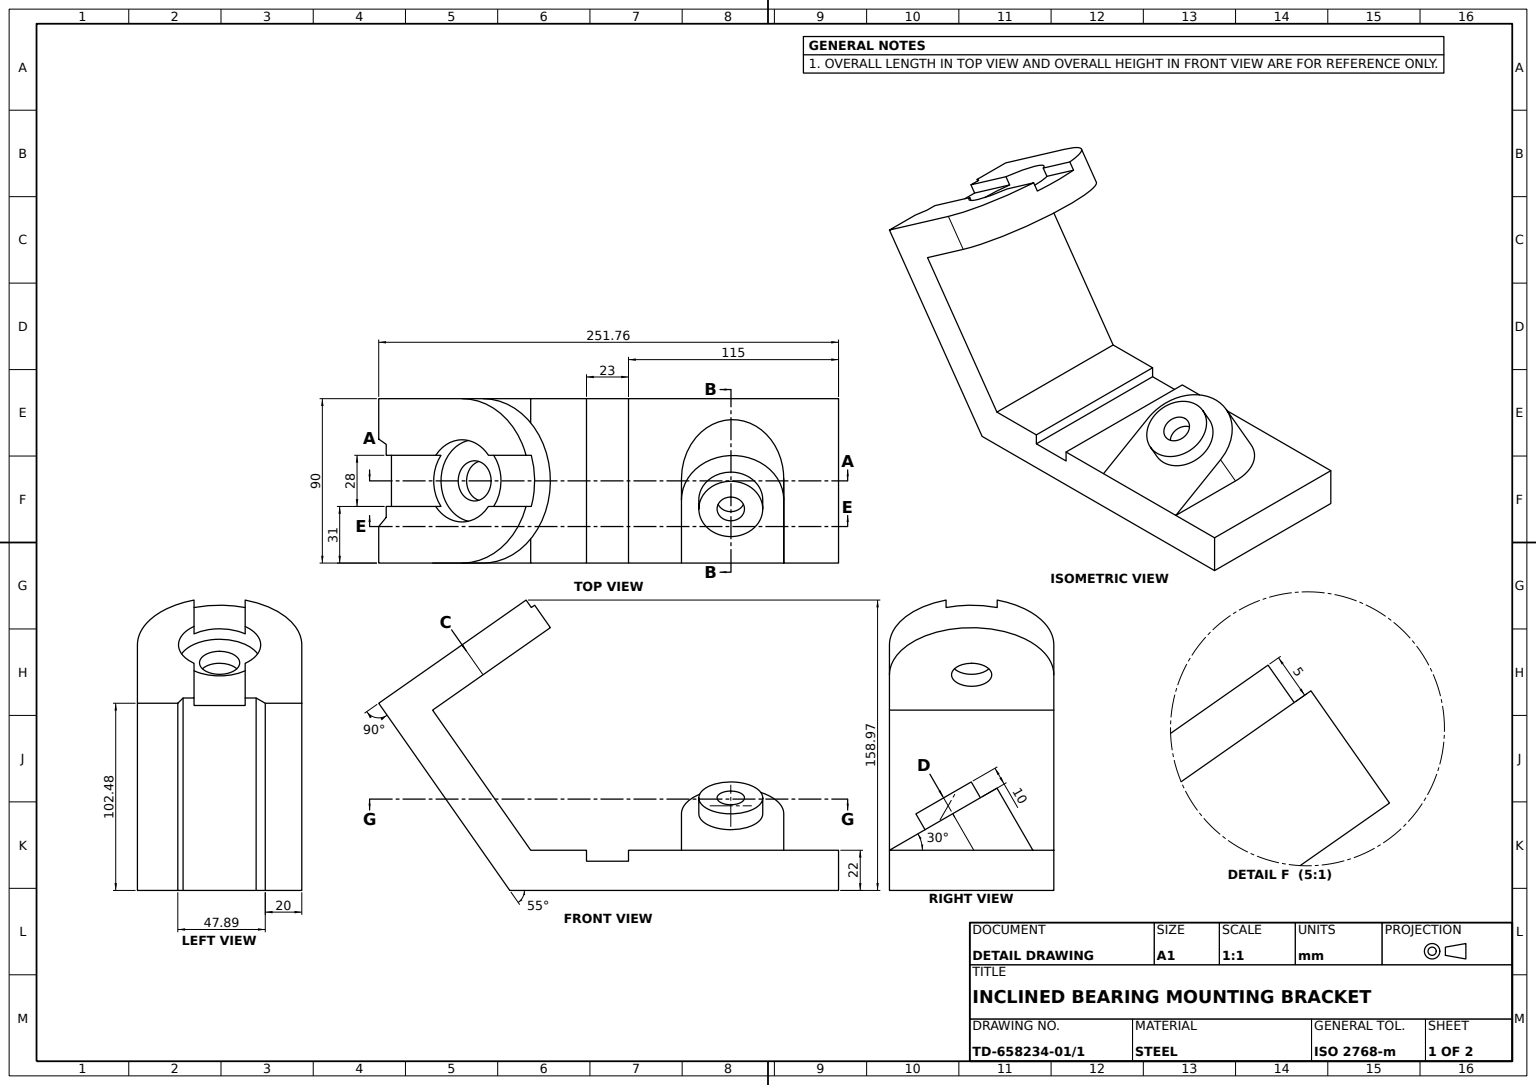
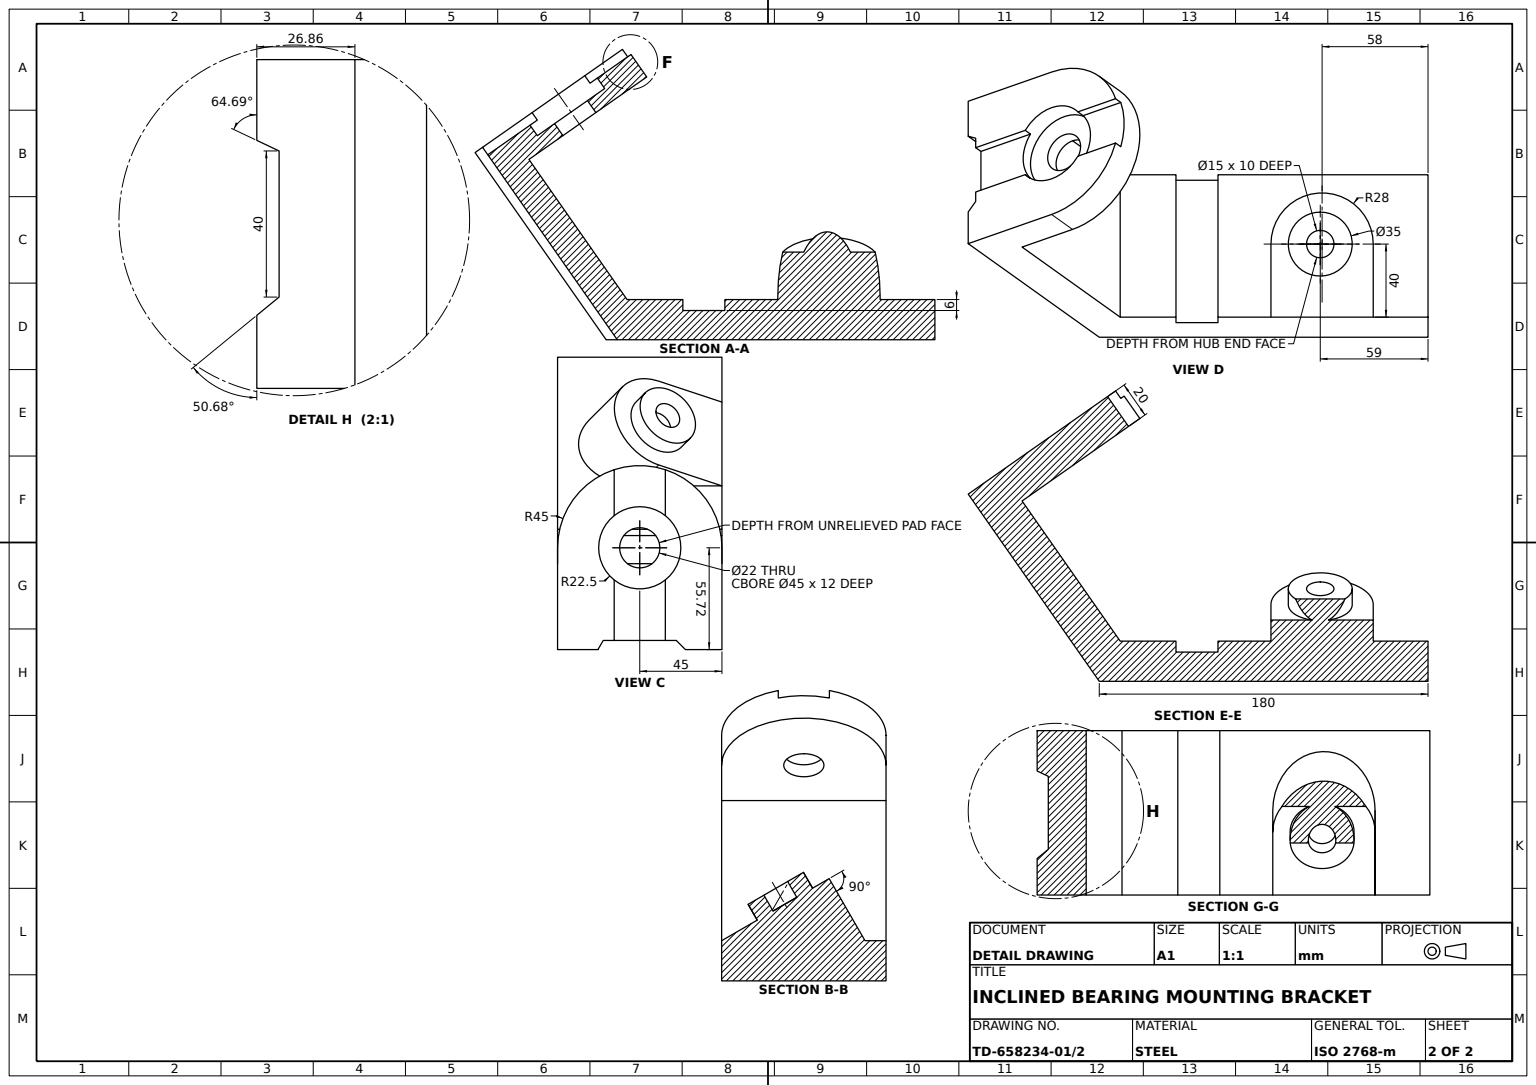
ISO-10303-21;
HEADER;
FILE_DESCRIPTION((''),'2;1');
FILE_NAME('','',(''),(''),'','','');
FILE_SCHEMA(('AUTOMOTIVE_DESIGN'));
ENDSEC;
DATA;
#1=APPLICATION_CONTEXT('');
#2=PRODUCT_CONTEXT('',#1,'mechanical');
#3=PRODUCT('','','',(#2));
#4=PRODUCT_DEFINITION_FORMATION('','',#3);
#5=PRODUCT_DEFINITION_CONTEXT('',#1,'design');
#6=PRODUCT_DEFINITION('','',#4,#5);
#7=PRODUCT_DEFINITION_SHAPE('','',#6);
#8=(LENGTH_UNIT()NAMED_UNIT(*)SI_UNIT(.MILLI.,.METRE.));
#9=(NAMED_UNIT(*)PLANE_ANGLE_UNIT()SI_UNIT($,.RADIAN.));
#10=(NAMED_UNIT(*)SI_UNIT($,.STERADIAN.)SOLID_ANGLE_UNIT());
#11=UNCERTAINTY_MEASURE_WITH_UNIT(LENGTH_MEASURE(0.005),#8,'distance_accuracy_value','');
#12=(GEOMETRIC_REPRESENTATION_CONTEXT(3)GLOBAL_UNCERTAINTY_ASSIGNED_CONTEXT((#11))GLOBAL_UNIT_ASSIGNED_CONTEXT((#8,#9,#10))REPRESENTATION_CONTEXT('',''));
#13=CARTESIAN_POINT('',(-1.188022,4.,22.));
#14=VERTEX_POINT('',#13);
#15=CARTESIAN_POINT('',(10.358984,4.,42.));
#16=VERTEX_POINT('',#15);
#17=CARTESIAN_POINT('',(-22.141016,4.,-14.291651));
#18=DIRECTION('',(0.5,0.,0.866025404));
#19=VECTOR('',#18,1000.);
#20=LINE('',#17,#19);
#21=EDGE_CURVE('',#14,#16,#20,.T.);
#22=ORIENTED_EDGE('',*,*,#21,.T.);
#23=CARTESIAN_POINT('',(10.358984,60.,42.));
#24=VERTEX_POINT('',#23);
#25=CARTESIAN_POINT('',(10.358984,32.,42.));
#26=DIRECTION('',(-0.866025404,0.,0.5));
#27=AXIS2_PLACEMENT_3D('',#25,#18,#26);
#28=CIRCLE('',#27,28.);
#29=EDGE_CURVE('',#24,#16,#28,.T.);
#30=ORIENTED_EDGE('',*,*,#29,.F.);
#31=CARTESIAN_POINT('',(-1.188022,60.,22.));
#32=VERTEX_POINT('',#31);
#33=CARTESIAN_POINT('',(-22.141016,60.,-14.291651));
#34=LINE('',#33,#19);
#35=EDGE_CURVE('',#32,#24,#34,.T.);
#36=ORIENTED_EDGE('',*,*,#35,.F.);
#37=CARTESIAN_POINT('',(-1.188022,32.,22.));
#38=DIRECTION('',(0.,0.,-1.));
#39=DIRECTION('',(1.,0.,0.));
#40=AXIS2_PLACEMENT_3D('',#37,#38,#39);
#41=ELLIPSE('',#40,32.331615,28.);
#42=EDGE_CURVE('',#14,#32,#41,.T.);
#43=ORIENTED_EDGE('',*,*,#42,.F.);
#44=EDGE_LOOP('',(#22,#30,#36,#43));
#45=FACE_BOUND('',#44,.T.);
#46=CARTESIAN_POINT('',(-22.141016,32.,-14.291651));
#47=DIRECTION('',(0.866025404,0.,-0.5));
#48=AXIS2_PLACEMENT_3D('',#46,#18,#47);
#49=CYLINDRICAL_SURFACE('',#48,28.);
#50=ADVANCED_FACE('',(#45),#49,.T.);
#51=CARTESIAN_POINT('',(3.863793,31.,45.75));
#52=VERTEX_POINT('',#51);
#53=CARTESIAN_POINT('',(10.358984,31.,42.));
#54=DIRECTION('',(-0.5,0.,-0.866025404));
#55=AXIS2_PLACEMENT_3D('',#53,#54,#26);
#56=CIRCLE('',#55,7.5);
#57=EDGE_CURVE('',#52,#52,#56,.F.);
#58=ORIENTED_EDGE('',*,*,#57,.T.);
#59=EDGE_LOOP('',(#58));
#60=FACE_BOUND('',#59,.T.);
#61=PLANE('',#55);
#62=ADVANCED_FACE('',(#60),#61,.F.);
#63=CARTESIAN_POINT('',(14.,-130.539677,124.339013));
#64=VERTEX_POINT('',#63);
#65=CARTESIAN_POINT('',(14.,-157.661612,105.34803));
#66=VERTEX_POINT('',#65);
#67=CARTESIAN_POINT('',(14.,-116.111202,134.44194));
#68=DIRECTION('',(0.,-0.819152044,-0.573576436));
#69=VECTOR('',#68,1000.);
#70=LINE('',#67,#69);
#71=EDGE_CURVE('',#64,#66,#70,.T.);
#72=ORIENTED_EDGE('',*,*,#71,.T.);
#73=CARTESIAN_POINT('',(20.,-157.661612,105.34803));
#74=VERTEX_POINT('',#73);
#75=CARTESIAN_POINT('',(0.,-157.661612,105.34803));
#76=DIRECTION('',(-1.,0.,0.));
#77=VECTOR('',#76,1000.);
#78=LINE('',#75,#77);
#79=EDGE_CURVE('',#74,#66,#78,.T.);
#80=ORIENTED_EDGE('',*,*,#79,.F.);
#81=CARTESIAN_POINT('',(25.,-161.757372,102.480148));
#82=VERTEX_POINT('',#81);
#83=DIRECTION('',(-0.707106781,0.579227965,0.405579788));
#84=VECTOR('',#83,1000.);
#85=LINE('',#81,#84);
#86=EDGE_CURVE('',#74,#82,#85,.F.);
#87=ORIENTED_EDGE('',*,*,#86,.T.);
#88=CARTESIAN_POINT('',(45.,-161.757372,102.480148));
#89=VERTEX_POINT('',#88);
#90=LINE('',#88,#77);
#91=EDGE_CURVE('',#82,#89,#90,.F.);
#92=ORIENTED_EDGE('',*,*,#91,.T.);
#93=CARTESIAN_POINT('',(45.,-116.111202,134.44194));
#94=VERTEX_POINT('',#93);
#95=LINE('',#93,#69);
#96=EDGE_CURVE('',#89,#94,#95,.F.);
#97=ORIENTED_EDGE('',*,*,#96,.T.);
#98=CARTESIAN_POINT('',(14.,-81.078683,158.971974));
#99=VERTEX_POINT('',#98);
#100=CARTESIAN_POINT('',(0.,-116.111202,134.44194));
#101=DIRECTION('',(0.,0.573576436,-0.819152044));
#102=AXIS2_PLACEMENT_3D('',#100,#101,#39);
#103=CIRCLE('',#102,45.);
#104=EDGE_CURVE('',#99,#94,#103,.T.);
#105=ORIENTED_EDGE('',*,*,#104,.F.);
#106=CARTESIAN_POINT('',(14.,-101.682728,144.544866));
#107=VERTEX_POINT('',#106);
#108=EDGE_CURVE('',#99,#107,#70,.T.);
#109=ORIENTED_EDGE('',*,*,#108,.T.);
#110=DIRECTION('',(0.,0.819152044,0.573576436));
#111=AXIS2_PLACEMENT_3D('',#100,#101,#110);
#112=CIRCLE('',#111,22.5);
#113=EDGE_CURVE('',#107,#64,#112,.T.);
#114=ORIENTED_EDGE('',*,*,#113,.T.);
#115=EDGE_LOOP('',(#72,#80,#87,#92,#97,#105,#109,#114));
#116=FACE_BOUND('',#115,.T.);
#117=PLANE('',#111);
#118=ADVANCED_FACE('',(#116),#117,.F.);
#119=CARTESIAN_POINT('',(0.203539,31.,59.410254));
#120=VERTEX_POINT('',#119);
#121=CARTESIAN_POINT('',(15.358984,31.,50.660254));
#122=AXIS2_PLACEMENT_3D('',#121,#18,#26);
#123=CIRCLE('',#122,17.5);
#124=EDGE_CURVE('',#120,#120,#123,.T.);
#125=ORIENTED_EDGE('',*,*,#124,.T.);
#126=EDGE_LOOP('',(#125));
#127=FACE_BOUND('',#126,.T.);
#128=CARTESIAN_POINT('',(8.863793,31.,54.410254));
#129=VERTEX_POINT('',#128);
#130=AXIS2_PLACEMENT_3D('',#121,#54,#26);
#131=CIRCLE('',#130,7.5);
#132=EDGE_CURVE('',#129,#129,#131,.T.);
#133=ORIENTED_EDGE('',*,*,#132,.T.);
#134=EDGE_LOOP('',(#133));
#135=FACE_BOUND('',#134,.T.);
#136=AXIS2_PLACEMENT_3D('',#121,#18,#47);
#137=PLANE('',#136);
#138=ADVANCED_FACE('',(#127,#135),#137,.T.);
#139=CARTESIAN_POINT('',(45.,-25.,16.));
#140=VERTEX_POINT('',#139);
#141=CARTESIAN_POINT('',(-45.,-25.,16.));
#142=VERTEX_POINT('',#141);
#143=CARTESIAN_POINT('',(-73.181818,-25.,16.));
#144=VECTOR('',#39,1000.);
#145=LINE('',#143,#144);
#146=EDGE_CURVE('',#140,#142,#145,.F.);
#147=ORIENTED_EDGE('',*,*,#146,.F.);
#148=CARTESIAN_POINT('',(45.,-25.,22.));
#149=VERTEX_POINT('',#148);
#150=CARTESIAN_POINT('',(45.,-25.,0.));
#151=DIRECTION('',(0.,0.,1.));
#152=VECTOR('',#151,1000.);
#153=LINE('',#150,#152);
#154=EDGE_CURVE('',#140,#149,#153,.T.);
#155=ORIENTED_EDGE('',*,*,#154,.T.);
#156=CARTESIAN_POINT('',(-45.,-25.,22.));
#157=VERTEX_POINT('',#156);
#158=LINE('',#148,#144);
#159=EDGE_CURVE('',#157,#149,#158,.T.);
#160=ORIENTED_EDGE('',*,*,#159,.F.);
#161=CARTESIAN_POINT('',(-45.,-25.,0.));
#162=LINE('',#161,#152);
#163=EDGE_CURVE('',#142,#157,#162,.T.);
#164=ORIENTED_EDGE('',*,*,#163,.F.);
#165=EDGE_LOOP('',(#147,#155,#160,#164));
#166=FACE_BOUND('',#165,.T.);
#167=CARTESIAN_POINT('',(-73.181818,-25.,48.));
#168=DIRECTION('',(0.,1.,0.));
#169=AXIS2_PLACEMENT_3D('',#167,#168,#151);
#170=PLANE('',#169);
#171=ADVANCED_FACE('',(#166),#170,.F.);
#172=ORIENTED_EDGE('',*,*,#71,.F.);
#173=CARTESIAN_POINT('',(14.,-127.671794,120.243253));
#174=VERTEX_POINT('',#173);
#175=VECTOR('',#101,1000.);
#176=LINE('',#63,#175);
#177=EDGE_CURVE('',#174,#64,#176,.F.);
#178=ORIENTED_EDGE('',*,*,#177,.F.);
#179=CARTESIAN_POINT('',(14.,-154.793729,101.252269));
#180=VERTEX_POINT('',#179);
#181=CARTESIAN_POINT('',(14.,-71.13713,159.829251));
#182=LINE('',#181,#69);
#183=EDGE_CURVE('',#180,#174,#182,.F.);
#184=ORIENTED_EDGE('',*,*,#183,.F.);
#185=CARTESIAN_POINT('',(14.,-180.031093,137.294959));
#186=LINE('',#185,#175);
#187=EDGE_CURVE('',#66,#180,#186,.T.);
#188=ORIENTED_EDGE('',*,*,#187,.F.);
#189=EDGE_LOOP('',(#172,#178,#184,#188));
#190=FACE_BOUND('',#189,.T.);
#191=CARTESIAN_POINT('',(14.,-96.374493,195.871941));
#192=AXIS2_PLACEMENT_3D('',#191,#39,#38);
#193=PLANE('',#192);
#194=ADVANCED_FACE('',(#190),#193,.F.);
#195=CARTESIAN_POINT('',(-45.,-161.757372,102.480148));
#196=VERTEX_POINT('',#195);
#197=CARTESIAN_POINT('',(-45.,-90.,0.));
#198=VERTEX_POINT('',#197);
#199=CARTESIAN_POINT('',(-45.,-161.697055,102.394006));
#200=LINE('',#199,#175);
#201=EDGE_CURVE('',#196,#198,#200,.T.);
#202=ORIENTED_EDGE('',*,*,#201,.T.);
#203=CARTESIAN_POINT('',(-22.886751,-90.,0.));
#204=VERTEX_POINT('',#203);
#205=CARTESIAN_POINT('',(45.,-90.,0.));
#206=LINE('',#205,#77);
#207=EDGE_CURVE('',#204,#198,#206,.T.);
#208=ORIENTED_EDGE('',*,*,#207,.F.);
#209=CARTESIAN_POINT('',(-22.886751,-161.757372,102.480148));
#210=VERTEX_POINT('',#209);
#211=DIRECTION('',(0.,-0.573576436,0.819152044));
#212=VECTOR('',#211,1000.);
#213=LINE('',#209,#212);
#214=EDGE_CURVE('',#204,#210,#213,.T.);
#215=ORIENTED_EDGE('',*,*,#214,.T.);
#216=EDGE_CURVE('',#196,#210,#90,.F.);
#217=ORIENTED_EDGE('',*,*,#216,.F.);
#218=EDGE_LOOP('',(#202,#208,#215,#217));
#219=FACE_BOUND('',#218,.T.);
#220=CARTESIAN_POINT('',(45.,-161.697055,102.394006));
#221=AXIS2_PLACEMENT_3D('',#220,#110,#211);
#222=PLANE('',#221);
#223=ADVANCED_FACE('',(#219),#222,.F.);
#224=CARTESIAN_POINT('',(-45.,90.,22.));
#225=VERTEX_POINT('',#224);
#226=DIRECTION('',(0.,-1.,0.));
#227=VECTOR('',#226,1000.);
#228=LINE('',#224,#227);
#229=EDGE_CURVE('',#225,#157,#228,.T.);
#230=ORIENTED_EDGE('',*,*,#229,.F.);
#231=CARTESIAN_POINT('',(-45.,90.,0.));
#232=VERTEX_POINT('',#231);
#233=LINE('',#231,#152);
#234=EDGE_CURVE('',#232,#225,#233,.T.);
#235=ORIENTED_EDGE('',*,*,#234,.F.);
#236=VECTOR('',#168,1000.);
#237=LINE('',#197,#236);
#238=EDGE_CURVE('',#198,#232,#237,.T.);
#239=ORIENTED_EDGE('',*,*,#238,.F.);
#240=ORIENTED_EDGE('',*,*,#201,.F.);
#241=CARTESIAN_POINT('',(-45.,-116.111202,134.44194));
#242=VERTEX_POINT('',#241);
#243=VECTOR('',#110,1000.);
#244=LINE('',#195,#243);
#245=EDGE_CURVE('',#242,#196,#244,.F.);
#246=ORIENTED_EDGE('',*,*,#245,.F.);
#247=CARTESIAN_POINT('',(-45.,-104.639673,118.058899));
#248=VERTEX_POINT('',#247);
#249=LINE('',#241,#175);
#250=EDGE_CURVE('',#248,#242,#249,.F.);
#251=ORIENTED_EDGE('',*,*,#250,.F.);
#252=CARTESIAN_POINT('',(-45.,-132.264498,98.715788));
#253=VERTEX_POINT('',#252);
#254=CARTESIAN_POINT('',(-45.,-150.285843,86.097107));
#255=LINE('',#254,#243);
#256=EDGE_CURVE('',#248,#253,#255,.F.);
#257=ORIENTED_EDGE('',*,*,#256,.T.);
#258=CARTESIAN_POINT('',(-45.,-78.547525,22.));
#259=VERTEX_POINT('',#258);
#260=CARTESIAN_POINT('',(-45.,-63.142959,0.));
#261=LINE('',#260,#212);
#262=EDGE_CURVE('',#259,#253,#261,.T.);
#263=ORIENTED_EDGE('',*,*,#262,.F.);
#264=CARTESIAN_POINT('',(-45.,-48.,22.));
#265=VERTEX_POINT('',#264);
#266=EDGE_CURVE('',#265,#259,#228,.T.);
#267=ORIENTED_EDGE('',*,*,#266,.F.);
#268=CARTESIAN_POINT('',(-45.,-48.,16.));
#269=VERTEX_POINT('',#268);
#270=CARTESIAN_POINT('',(-45.,-48.,0.));
#271=VECTOR('',#38,1000.);
#272=LINE('',#270,#271);
#273=EDGE_CURVE('',#265,#269,#272,.T.);
#274=ORIENTED_EDGE('',*,*,#273,.T.);
#275=CARTESIAN_POINT('',(-45.,0.,16.));
#276=LINE('',#275,#236);
#277=EDGE_CURVE('',#269,#142,#276,.T.);
#278=ORIENTED_EDGE('',*,*,#277,.T.);
#279=ORIENTED_EDGE('',*,*,#163,.T.);
#280=EDGE_LOOP('',(#230,#235,#239,#240,#246,#251,#257,#263,#267,#274,#278,#279));
#281=FACE_BOUND('',#280,.T.);
#282=CARTESIAN_POINT('',(-45.,0.,0.));
#283=AXIS2_PLACEMENT_3D('',#282,#39,#38);
#284=PLANE('',#283);
#285=ADVANCED_FACE('',(#281),#284,.F.);
#286=CARTESIAN_POINT('',(-14.,-81.078683,158.971974));
#287=VERTEX_POINT('',#286);
#288=EDGE_CURVE('',#242,#287,#103,.T.);
#289=ORIENTED_EDGE('',*,*,#288,.F.);
#290=ORIENTED_EDGE('',*,*,#245,.T.);
#291=ORIENTED_EDGE('',*,*,#216,.T.);
#292=CARTESIAN_POINT('',(-20.,-157.661612,105.34803));
#293=VERTEX_POINT('',#292);
#294=DIRECTION('',(0.5,0.70940648,0.496731765));
#295=VECTOR('',#294,1000.);
#296=LINE('',#292,#295);
#297=EDGE_CURVE('',#210,#293,#296,.T.);
#298=ORIENTED_EDGE('',*,*,#297,.T.);
#299=CARTESIAN_POINT('',(-14.,-157.661612,105.34803));
#300=VERTEX_POINT('',#299);
#301=EDGE_CURVE('',#300,#293,#78,.T.);
#302=ORIENTED_EDGE('',*,*,#301,.F.);
#303=CARTESIAN_POINT('',(-14.,-130.539677,124.339013));
#304=VERTEX_POINT('',#303);
#305=CARTESIAN_POINT('',(-14.,-116.111202,134.44194));
#306=LINE('',#305,#243);
#307=EDGE_CURVE('',#300,#304,#306,.T.);
#308=ORIENTED_EDGE('',*,*,#307,.T.);
#309=CARTESIAN_POINT('',(-14.,-101.682728,144.544866));
#310=VERTEX_POINT('',#309);
#311=EDGE_CURVE('',#304,#310,#112,.T.);
#312=ORIENTED_EDGE('',*,*,#311,.T.);
#313=EDGE_CURVE('',#310,#287,#306,.T.);
#314=ORIENTED_EDGE('',*,*,#313,.T.);
#315=EDGE_LOOP('',(#289,#290,#291,#298,#302,#308,#312,#314));
#316=FACE_BOUND('',#315,.T.);
#317=ADVANCED_FACE('',(#316),#117,.F.);
#318=ORIENTED_EDGE('',*,*,#35,.T.);
#319=CARTESIAN_POINT('',(45.,60.,22.));
#320=VERTEX_POINT('',#319);
#321=CARTESIAN_POINT('',(52.566069,60.,17.631728));
#322=VECTOR('',#26,1000.);
#323=LINE('',#321,#322);
#324=EDGE_CURVE('',#320,#24,#323,.T.);
#325=ORIENTED_EDGE('',*,*,#324,.F.);
#326=LINE('',#319,#144);
#327=EDGE_CURVE('',#32,#320,#326,.T.);
#328=ORIENTED_EDGE('',*,*,#327,.F.);
#329=EDGE_LOOP('',(#318,#325,#328));
#330=FACE_BOUND('',#329,.T.);
#331=CARTESIAN_POINT('',(20.066069,60.,-38.659923));
#332=AXIS2_PLACEMENT_3D('',#331,#168,#76);
#333=PLANE('',#332);
#334=ADVANCED_FACE('',(#330),#333,.T.);
#335=ORIENTED_EDGE('',*,*,#183,.T.);
#336=CARTESIAN_POINT('',(-14.,-127.671794,120.243253));
#337=VERTEX_POINT('',#336);
#338=CARTESIAN_POINT('',(0.,-113.24332,130.346179));
#339=AXIS2_PLACEMENT_3D('',#338,#101,#110);
#340=CIRCLE('',#339,22.5);
#341=EDGE_CURVE('',#337,#174,#340,.F.);
#342=ORIENTED_EDGE('',*,*,#341,.F.);
#343=CARTESIAN_POINT('',(-14.,-154.793729,101.252269));
#344=VERTEX_POINT('',#343);
#345=CARTESIAN_POINT('',(-14.,-202.893985,67.572108));
#346=LINE('',#345,#243);
#347=EDGE_CURVE('',#337,#344,#346,.F.);
#348=ORIENTED_EDGE('',*,*,#347,.T.);
#349=CARTESIAN_POINT('',(0.,-154.793729,101.252269));
#350=LINE('',#349,#77);
#351=EDGE_CURVE('',#180,#344,#350,.T.);
#352=ORIENTED_EDGE('',*,*,#351,.F.);
#353=EDGE_LOOP('',(#335,#342,#348,#352));
#354=FACE_BOUND('',#353,.T.);
#355=CARTESIAN_POINT('',(0.,-98.498583,140.670555));
#356=AXIS2_PLACEMENT_3D('',#355,#101,#110);
#357=PLANE('',#356);
#358=ADVANCED_FACE('',(#354),#357,.F.);
#359=CARTESIAN_POINT('',(-20.,-83.896127,0.));
#360=VERTEX_POINT('',#359);
#361=CARTESIAN_POINT('',(20.,-83.896127,0.));
#362=VERTEX_POINT('',#361);
#363=LINE('',#361,#77);
#364=EDGE_CURVE('',#360,#362,#363,.F.);
#365=ORIENTED_EDGE('',*,*,#364,.F.);
#366=CARTESIAN_POINT('',(-9.332465,-61.340225,0.));
#367=DIRECTION('',(-0.427535057,-0.90399877,0.));
#368=VECTOR('',#367,1000.);
#369=LINE('',#366,#368);
#370=EDGE_CURVE('',#360,#204,#369,.T.);
#371=ORIENTED_EDGE('',*,*,#370,.T.);
#372=ORIENTED_EDGE('',*,*,#207,.T.);
#373=ORIENTED_EDGE('',*,*,#238,.T.);
#374=CARTESIAN_POINT('',(45.,90.,0.));
#375=VERTEX_POINT('',#374);
#376=LINE('',#374,#77);
#377=EDGE_CURVE('',#375,#232,#376,.T.);
#378=ORIENTED_EDGE('',*,*,#377,.F.);
#379=VERTEX_POINT('',#205);
#380=LINE('',#205,#236);
#381=EDGE_CURVE('',#379,#375,#380,.T.);
#382=ORIENTED_EDGE('',*,*,#381,.F.);
#383=CARTESIAN_POINT('',(25.,-90.,0.));
#384=VERTEX_POINT('',#383);
#385=EDGE_CURVE('',#379,#384,#206,.T.);
#386=ORIENTED_EDGE('',*,*,#385,.T.);
#387=CARTESIAN_POINT('',(60.146879,-132.906417,0.));
#388=DIRECTION('',(0.633687274,-0.773589322,0.));
#389=VECTOR('',#388,1000.);
#390=LINE('',#387,#389);
#391=EDGE_CURVE('',#384,#362,#390,.F.);
#392=ORIENTED_EDGE('',*,*,#391,.T.);
#393=EDGE_LOOP('',(#365,#371,#372,#373,#378,#382,#386,#392));
#394=FACE_BOUND('',#393,.T.);
#395=AXIS2_PLACEMENT_3D('',#205,#151,#39);
#396=PLANE('',#395);
#397=ADVANCED_FACE('',(#394),#396,.F.);
#398=ORIENTED_EDGE('',*,*,#301,.T.);
#399=LINE('',#359,#212);
#400=EDGE_CURVE('',#293,#360,#399,.F.);
#401=ORIENTED_EDGE('',*,*,#400,.T.);
#402=ORIENTED_EDGE('',*,*,#364,.T.);
#403=LINE('',#361,#212);
#404=EDGE_CURVE('',#74,#362,#403,.F.);
#405=ORIENTED_EDGE('',*,*,#404,.F.);
#406=ORIENTED_EDGE('',*,*,#79,.T.);
#407=ORIENTED_EDGE('',*,*,#187,.T.);
#408=ORIENTED_EDGE('',*,*,#351,.T.);
#409=CARTESIAN_POINT('',(-14.,-180.031093,137.294959));
#410=LINE('',#409,#212);
#411=EDGE_CURVE('',#344,#300,#410,.T.);
#412=ORIENTED_EDGE('',*,*,#411,.T.);
#413=EDGE_LOOP('',(#398,#401,#402,#405,#406,#407,#408,#412));
#414=FACE_BOUND('',#413,.T.);
#415=AXIS2_PLACEMENT_3D('',#361,#68,#101);
#416=PLANE('',#415);
#417=ADVANCED_FACE('',(#414),#416,.T.);
#418=CARTESIAN_POINT('',(14.,-78.210801,154.876214));
#419=VERTEX_POINT('',#418);
#420=LINE('',#98,#175);
#421=EDGE_CURVE('',#99,#419,#420,.T.);
#422=ORIENTED_EDGE('',*,*,#421,.T.);
#423=CARTESIAN_POINT('',(14.,-98.814846,140.449106));
#424=VERTEX_POINT('',#423);
#425=EDGE_CURVE('',#424,#419,#182,.F.);
#426=ORIENTED_EDGE('',*,*,#425,.F.);
#427=LINE('',#106,#175);
#428=EDGE_CURVE('',#107,#424,#427,.T.);
#429=ORIENTED_EDGE('',*,*,#428,.F.);
#430=ORIENTED_EDGE('',*,*,#108,.F.);
#431=EDGE_LOOP('',(#422,#426,#429,#430));
#432=FACE_BOUND('',#431,.T.);
#433=ADVANCED_FACE('',(#432),#193,.F.);
#434=CARTESIAN_POINT('',(45.,-78.547525,22.));
#435=VERTEX_POINT('',#434);
#436=LINE('',#434,#77);
#437=EDGE_CURVE('',#435,#259,#436,.T.);
#438=ORIENTED_EDGE('',*,*,#437,.F.);
#439=CARTESIAN_POINT('',(45.,-48.,22.));
#440=VERTEX_POINT('',#439);
#441=CARTESIAN_POINT('',(45.,90.,22.));
#442=LINE('',#441,#227);
#443=EDGE_CURVE('',#440,#435,#442,.T.);
#444=ORIENTED_EDGE('',*,*,#443,.F.);
#445=LINE('',#439,#77);
#446=EDGE_CURVE('',#440,#265,#445,.T.);
#447=ORIENTED_EDGE('',*,*,#446,.T.);
#448=ORIENTED_EDGE('',*,*,#266,.T.);
#449=EDGE_LOOP('',(#438,#444,#447,#448));
#450=FACE_BOUND('',#449,.T.);
#451=AXIS2_PLACEMENT_3D('',#441,#38,#76);
#452=PLANE('',#451);
#453=ADVANCED_FACE('',(#450),#452,.F.);
#454=ORIENTED_EDGE('',*,*,#391,.F.);
#455=CARTESIAN_POINT('',(25.,-161.697055,102.394006));
#456=LINE('',#455,#175);
#457=EDGE_CURVE('',#82,#384,#456,.T.);
#458=ORIENTED_EDGE('',*,*,#457,.F.);
#459=ORIENTED_EDGE('',*,*,#86,.F.);
#460=ORIENTED_EDGE('',*,*,#404,.T.);
#461=EDGE_LOOP('',(#454,#458,#459,#460));
#462=FACE_BOUND('',#461,.T.);
#463=DIRECTION('',(0.707106781,0.579227965,0.405579788));
#464=AXIS2_PLACEMENT_3D('',#455,#463,#101);
#465=PLANE('',#464);
#466=ADVANCED_FACE('',(#462),#465,.F.);
#467=CARTESIAN_POINT('',(0.,-90.797364,137.517585));
#468=VERTEX_POINT('',#467);
#469=CARTESIAN_POINT('',(0.,-109.228285,124.612115));
#470=AXIS2_PLACEMENT_3D('',#469,#101,#110);
#471=CIRCLE('',#470,22.5);
#472=EDGE_CURVE('',#468,#468,#471,.F.);
#473=ORIENTED_EDGE('',*,*,#472,.F.);
#474=EDGE_LOOP('',(#473));
#475=FACE_BOUND('',#474,.T.);
#476=ORIENTED_EDGE('',*,*,#311,.F.);
#477=LINE('',#303,#175);
#478=EDGE_CURVE('',#304,#337,#477,.T.);
#479=ORIENTED_EDGE('',*,*,#478,.T.);
#480=ORIENTED_EDGE('',*,*,#341,.T.);
#481=ORIENTED_EDGE('',*,*,#177,.T.);
#482=ORIENTED_EDGE('',*,*,#113,.F.);
#483=ORIENTED_EDGE('',*,*,#428,.T.);
#484=CARTESIAN_POINT('',(-14.,-98.814846,140.449106));
#485=VERTEX_POINT('',#484);
#486=EDGE_CURVE('',#424,#485,#340,.F.);
#487=ORIENTED_EDGE('',*,*,#486,.T.);
#488=LINE('',#309,#175);
#489=EDGE_CURVE('',#485,#310,#488,.F.);
#490=ORIENTED_EDGE('',*,*,#489,.T.);
#491=EDGE_LOOP('',(#476,#479,#480,#481,#482,#483,#487,#490));
#492=FACE_BOUND('',#491,.T.);
#493=CYLINDRICAL_SURFACE('',#111,22.5);
#494=ADVANCED_FACE('',(#475,#492),#493,.F.);
#495=ORIENTED_EDGE('',*,*,#400,.F.);
#496=ORIENTED_EDGE('',*,*,#297,.F.);
#497=ORIENTED_EDGE('',*,*,#214,.F.);
#498=ORIENTED_EDGE('',*,*,#370,.F.);
#499=EDGE_LOOP('',(#495,#496,#497,#498));
#500=FACE_BOUND('',#499,.T.);
#501=CARTESIAN_POINT('',(-20.,-56.295146,-39.418286));
#502=DIRECTION('',(0.866025404,-0.409576022,-0.286788218));
#503=AXIS2_PLACEMENT_3D('',#501,#502,#211);
#504=PLANE('',#503);
#505=ADVANCED_FACE('',(#500),#504,.T.);
#506=ORIENTED_EDGE('',*,*,#425,.T.);
#507=CARTESIAN_POINT('',(-14.,-78.210801,154.876214));
#508=VERTEX_POINT('',#507);
#509=CIRCLE('',#339,45.);
#510=EDGE_CURVE('',#419,#508,#509,.F.);
#511=ORIENTED_EDGE('',*,*,#510,.T.);
#512=EDGE_CURVE('',#508,#485,#346,.F.);
#513=ORIENTED_EDGE('',*,*,#512,.T.);
#514=ORIENTED_EDGE('',*,*,#486,.F.);
#515=EDGE_LOOP('',(#506,#511,#513,#514));
#516=FACE_BOUND('',#515,.T.);
#517=ADVANCED_FACE('',(#516),#357,.F.);
#518=ORIENTED_EDGE('',*,*,#91,.F.);
#519=ORIENTED_EDGE('',*,*,#457,.T.);
#520=ORIENTED_EDGE('',*,*,#385,.F.);
#521=LINE('',#220,#175);
#522=EDGE_CURVE('',#89,#379,#521,.T.);
#523=ORIENTED_EDGE('',*,*,#522,.F.);
#524=EDGE_LOOP('',(#518,#519,#520,#523));
#525=FACE_BOUND('',#524,.T.);
#526=ADVANCED_FACE('',(#525),#222,.F.);
#527=CARTESIAN_POINT('',(45.,-104.639673,118.058899));
#528=VERTEX_POINT('',#527);
#529=CARTESIAN_POINT('',(0.,-104.639673,118.058899));
#530=AXIS2_PLACEMENT_3D('',#529,#101,#39);
#531=CIRCLE('',#530,45.);
#532=EDGE_CURVE('',#248,#528,#531,.T.);
#533=ORIENTED_EDGE('',*,*,#532,.F.);
#534=ORIENTED_EDGE('',*,*,#250,.T.);
#535=ORIENTED_EDGE('',*,*,#288,.T.);
#536=LINE('',#286,#175);
#537=EDGE_CURVE('',#508,#287,#536,.F.);
#538=ORIENTED_EDGE('',*,*,#537,.F.);
#539=ORIENTED_EDGE('',*,*,#510,.F.);
#540=ORIENTED_EDGE('',*,*,#421,.F.);
#541=ORIENTED_EDGE('',*,*,#104,.T.);
#542=LINE('',#93,#175);
#543=EDGE_CURVE('',#528,#94,#542,.F.);
#544=ORIENTED_EDGE('',*,*,#543,.F.);
#545=EDGE_LOOP('',(#533,#534,#535,#538,#539,#540,#541,#544));
#546=FACE_BOUND('',#545,.T.);
#547=CYLINDRICAL_SURFACE('',#111,45.);
#548=ADVANCED_FACE('',(#546),#547,.T.);
#549=ORIENTED_EDGE('',*,*,#411,.F.);
#550=ORIENTED_EDGE('',*,*,#347,.F.);
#551=ORIENTED_EDGE('',*,*,#478,.F.);
#552=ORIENTED_EDGE('',*,*,#307,.F.);
#553=EDGE_LOOP('',(#549,#550,#551,#552));
#554=FACE_BOUND('',#553,.T.);
#555=CARTESIAN_POINT('',(-14.,-228.131348,103.614798));
#556=AXIS2_PLACEMENT_3D('',#555,#76,#151);
#557=PLANE('',#556);
#558=ADVANCED_FACE('',(#554),#557,.F.);
#559=ORIENTED_EDGE('',*,*,#21,.F.);
#560=CARTESIAN_POINT('',(45.,4.,22.));
#561=VERTEX_POINT('',#560);
#562=LINE('',#560,#77);
#563=EDGE_CURVE('',#561,#14,#562,.T.);
#564=ORIENTED_EDGE('',*,*,#563,.F.);
#565=VECTOR('',#47,1000.);
#566=LINE('',#15,#565);
#567=EDGE_CURVE('',#16,#561,#566,.T.);
#568=ORIENTED_EDGE('',*,*,#567,.F.);
#569=EDGE_LOOP('',(#559,#564,#568));
#570=FACE_BOUND('',#569,.T.);
#571=AXIS2_PLACEMENT_3D('',#17,#226,#39);
#572=PLANE('',#571);
#573=ADVANCED_FACE('',(#570),#572,.T.);
#574=ORIENTED_EDGE('',*,*,#472,.T.);
#575=EDGE_LOOP('',(#574));
#576=FACE_BOUND('',#575,.T.);
#577=CARTESIAN_POINT('',(0.,-100.217612,130.921456));
#578=VERTEX_POINT('',#577);
#579=CIRCLE('',#470,11.);
#580=EDGE_CURVE('',#578,#578,#579,.F.);
#581=ORIENTED_EDGE('',*,*,#580,.F.);
#582=EDGE_LOOP('',(#581));
#583=FACE_BOUND('',#582,.T.);
#584=PLANE('',#470);
#585=ADVANCED_FACE('',(#576,#583),#584,.F.);
#586=ORIENTED_EDGE('',*,*,#381,.T.);
#587=VERTEX_POINT('',#441);
#588=LINE('',#374,#152);
#589=EDGE_CURVE('',#375,#587,#588,.T.);
#590=ORIENTED_EDGE('',*,*,#589,.T.);
#591=EDGE_CURVE('',#587,#320,#442,.T.);
#592=ORIENTED_EDGE('',*,*,#591,.T.);
#593=EDGE_CURVE('',#320,#561,#442,.T.);
#594=ORIENTED_EDGE('',*,*,#593,.T.);
#595=EDGE_CURVE('',#561,#149,#442,.T.);
#596=ORIENTED_EDGE('',*,*,#595,.T.);
#597=ORIENTED_EDGE('',*,*,#154,.F.);
#598=CARTESIAN_POINT('',(45.,-48.,16.));
#599=VERTEX_POINT('',#598);
#600=CARTESIAN_POINT('',(45.,0.,16.));
#601=LINE('',#600,#236);
#602=EDGE_CURVE('',#599,#140,#601,.T.);
#603=ORIENTED_EDGE('',*,*,#602,.F.);
#604=CARTESIAN_POINT('',(45.,-48.,0.));
#605=LINE('',#604,#271);
#606=EDGE_CURVE('',#440,#599,#605,.T.);
#607=ORIENTED_EDGE('',*,*,#606,.F.);
#608=ORIENTED_EDGE('',*,*,#443,.T.);
#609=CARTESIAN_POINT('',(45.,-132.264498,98.715788));
#610=VERTEX_POINT('',#609);
#611=CARTESIAN_POINT('',(45.,-63.142959,0.));
#612=LINE('',#611,#212);
#613=EDGE_CURVE('',#435,#610,#612,.T.);
#614=ORIENTED_EDGE('',*,*,#613,.T.);
#615=LINE('',#527,#69);
#616=EDGE_CURVE('',#610,#528,#615,.F.);
#617=ORIENTED_EDGE('',*,*,#616,.T.);
#618=ORIENTED_EDGE('',*,*,#543,.T.);
#619=ORIENTED_EDGE('',*,*,#96,.F.);
#620=ORIENTED_EDGE('',*,*,#522,.T.);
#621=EDGE_LOOP('',(#586,#590,#592,#594,#596,#597,#603,#607,#608,#614,#617,#618,#619,#620));
#622=FACE_BOUND('',#621,.T.);
#623=CARTESIAN_POINT('',(45.,0.,0.));
#624=AXIS2_PLACEMENT_3D('',#623,#39,#38);
#625=PLANE('',#624);
#626=ADVANCED_FACE('',(#622),#625,.T.);
#627=ORIENTED_EDGE('',*,*,#256,.F.);
#628=ORIENTED_EDGE('',*,*,#532,.T.);
#629=ORIENTED_EDGE('',*,*,#616,.F.);
#630=LINE('',#609,#144);
#631=EDGE_CURVE('',#253,#610,#630,.T.);
#632=ORIENTED_EDGE('',*,*,#631,.F.);
#633=EDGE_LOOP('',(#627,#628,#629,#632));
#634=FACE_BOUND('',#633,.T.);
#635=CARTESIAN_POINT('',(0.,-95.629001,124.36824));
#636=VERTEX_POINT('',#635);
#637=AXIS2_PLACEMENT_3D('',#529,#101,#110);
#638=CIRCLE('',#637,11.);
#639=EDGE_CURVE('',#636,#636,#638,.T.);
#640=ORIENTED_EDGE('',*,*,#639,.F.);
#641=EDGE_LOOP('',(#640));
#642=FACE_BOUND('',#641,.T.);
#643=PLANE('',#637);
#644=ADVANCED_FACE('',(#634,#642),#643,.T.);
#645=LINE('',#441,#77);
#646=EDGE_CURVE('',#587,#225,#645,.T.);
#647=ORIENTED_EDGE('',*,*,#646,.F.);
#648=ORIENTED_EDGE('',*,*,#589,.F.);
#649=ORIENTED_EDGE('',*,*,#377,.T.);
#650=ORIENTED_EDGE('',*,*,#234,.T.);
#651=EDGE_LOOP('',(#647,#648,#649,#650));
#652=FACE_BOUND('',#651,.T.);
#653=AXIS2_PLACEMENT_3D('',#374,#226,#38);
#654=PLANE('',#653);
#655=ADVANCED_FACE('',(#652),#654,.F.);
#656=ORIENTED_EDGE('',*,*,#327,.T.);
#657=ORIENTED_EDGE('',*,*,#591,.F.);
#658=ORIENTED_EDGE('',*,*,#646,.T.);
#659=ORIENTED_EDGE('',*,*,#229,.T.);
#660=ORIENTED_EDGE('',*,*,#159,.T.);
#661=ORIENTED_EDGE('',*,*,#595,.F.);
#662=ORIENTED_EDGE('',*,*,#563,.T.);
#663=ORIENTED_EDGE('',*,*,#42,.T.);
#664=EDGE_LOOP('',(#656,#657,#658,#659,#660,#661,#662,#663));
#665=FACE_BOUND('',#664,.T.);
#666=ADVANCED_FACE('',(#665),#452,.F.);
#667=ORIENTED_EDGE('',*,*,#580,.T.);
#668=EDGE_LOOP('',(#667));
#669=FACE_BOUND('',#668,.T.);
#670=ORIENTED_EDGE('',*,*,#639,.T.);
#671=EDGE_LOOP('',(#670));
#672=FACE_BOUND('',#671,.T.);
#673=CYLINDRICAL_SURFACE('',#637,11.);
#674=ADVANCED_FACE('',(#669,#672),#673,.F.);
#675=ORIENTED_EDGE('',*,*,#437,.T.);
#676=ORIENTED_EDGE('',*,*,#262,.T.);
#677=ORIENTED_EDGE('',*,*,#631,.T.);
#678=ORIENTED_EDGE('',*,*,#613,.F.);
#679=EDGE_LOOP('',(#675,#676,#677,#678));
#680=FACE_BOUND('',#679,.T.);
#681=AXIS2_PLACEMENT_3D('',#611,#68,#101);
#682=PLANE('',#681);
#683=ADVANCED_FACE('',(#680),#682,.F.);
#684=CARTESIAN_POINT('',(25.514428,31.,33.25));
#685=VERTEX_POINT('',#684);
#686=AXIS2_PLACEMENT_3D('',#53,#18,#47);
#687=CIRCLE('',#686,17.5);
#688=EDGE_CURVE('',#685,#685,#687,.F.);
#689=ORIENTED_EDGE('',*,*,#688,.F.);
#690=EDGE_LOOP('',(#689));
#691=FACE_BOUND('',#690,.T.);
#692=ORIENTED_EDGE('',*,*,#124,.F.);
#693=EDGE_LOOP('',(#692));
#694=FACE_BOUND('',#693,.T.);
#695=CYLINDRICAL_SURFACE('',#130,17.5);
#696=ADVANCED_FACE('',(#691,#694),#695,.T.);
#697=CARTESIAN_POINT('',(73.181818,-48.,16.));
#698=LINE('',#697,#77);
#699=EDGE_CURVE('',#269,#599,#698,.F.);
#700=ORIENTED_EDGE('',*,*,#699,.T.);
#701=ORIENTED_EDGE('',*,*,#602,.T.);
#702=ORIENTED_EDGE('',*,*,#146,.T.);
#703=ORIENTED_EDGE('',*,*,#277,.F.);
#704=EDGE_LOOP('',(#700,#701,#702,#703));
#705=FACE_BOUND('',#704,.T.);
#706=CARTESIAN_POINT('',(0.,0.,16.));
#707=AXIS2_PLACEMENT_3D('',#706,#38,#76);
#708=PLANE('',#707);
#709=ADVANCED_FACE('',(#705),#708,.F.);
#710=ORIENTED_EDGE('',*,*,#699,.F.);
#711=ORIENTED_EDGE('',*,*,#273,.F.);
#712=ORIENTED_EDGE('',*,*,#446,.F.);
#713=ORIENTED_EDGE('',*,*,#606,.T.);
#714=EDGE_LOOP('',(#710,#711,#712,#713));
#715=FACE_BOUND('',#714,.T.);
#716=CARTESIAN_POINT('',(73.181818,-48.,48.));
#717=AXIS2_PLACEMENT_3D('',#716,#226,#38);
#718=PLANE('',#717);
#719=ADVANCED_FACE('',(#715),#718,.F.);
#720=ORIENTED_EDGE('',*,*,#688,.T.);
#721=EDGE_LOOP('',(#720));
#722=FACE_BOUND('',#721,.T.);
#723=ORIENTED_EDGE('',*,*,#29,.T.);
#724=ORIENTED_EDGE('',*,*,#567,.T.);
#725=ORIENTED_EDGE('',*,*,#593,.F.);
#726=ORIENTED_EDGE('',*,*,#324,.T.);
#727=EDGE_LOOP('',(#723,#724,#725,#726));
#728=FACE_BOUND('',#727,.T.);
#729=AXIS2_PLACEMENT_3D('',#25,#18,#47);
#730=PLANE('',#729);
#731=ADVANCED_FACE('',(#722,#728),#730,.T.);
#732=ORIENTED_EDGE('',*,*,#57,.F.);
#733=EDGE_LOOP('',(#732));
#734=FACE_BOUND('',#733,.T.);
#735=ORIENTED_EDGE('',*,*,#132,.F.);
#736=EDGE_LOOP('',(#735));
#737=FACE_BOUND('',#736,.T.);
#738=CYLINDRICAL_SURFACE('',#130,7.5);
#739=ADVANCED_FACE('',(#734,#737),#738,.F.);
#740=ORIENTED_EDGE('',*,*,#489,.F.);
#741=ORIENTED_EDGE('',*,*,#512,.F.);
#742=ORIENTED_EDGE('',*,*,#537,.T.);
#743=ORIENTED_EDGE('',*,*,#313,.F.);
#744=EDGE_LOOP('',(#740,#741,#742,#743));
#745=FACE_BOUND('',#744,.T.);
#746=ADVANCED_FACE('',(#745),#557,.F.);
#747=CLOSED_SHELL('',(#50,#62,#118,#138,#171,#194,#223,#285,#317,#334,#358,#397,#417,#433,#453,#466,#494,#505,#517,#526,#548,#558,#573,#585,#626,#644,#655,#666,#674,#683,#696,#709,#719,#731,#739,#746));
#748=MANIFOLD_SOLID_BREP('',#747);
#749=ADVANCED_BREP_SHAPE_REPRESENTATION('',(#748),#12);
#750=SHAPE_DEFINITION_REPRESENTATION(#7,#749);
ENDSEC;
END-ISO-10303-21;
